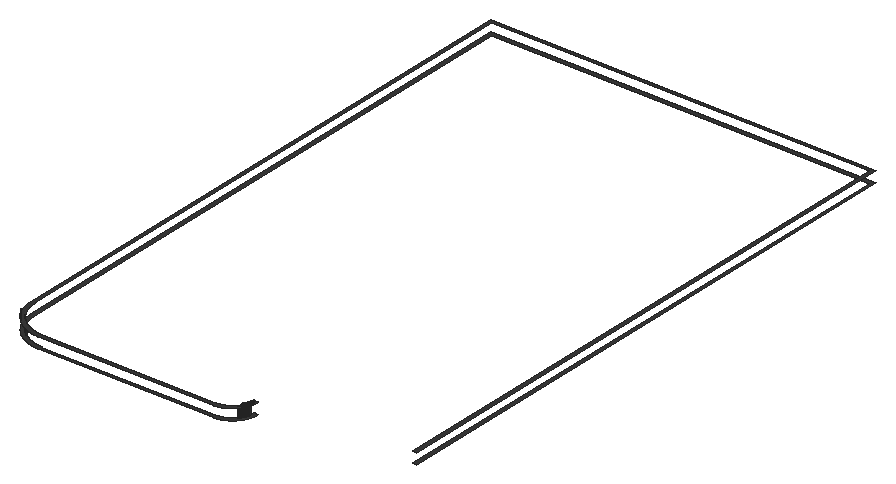
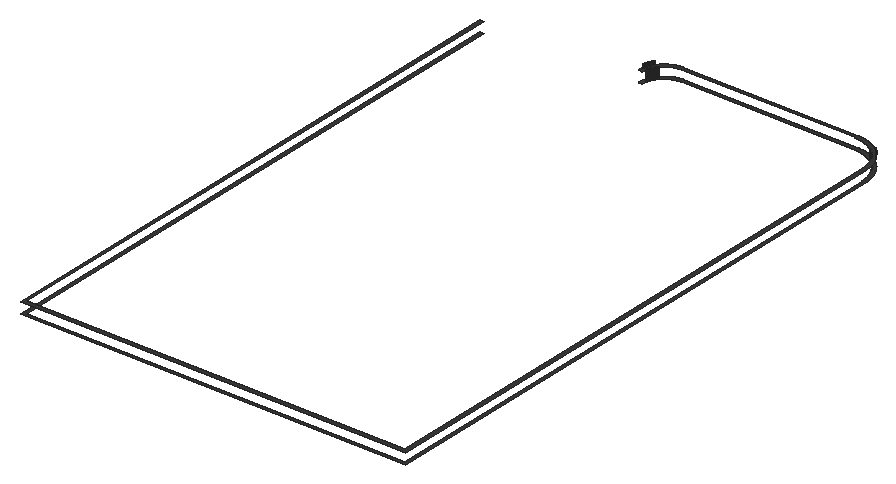
# SketchUp Ruby script. Lengths in inches.
U = 1.inch
M = Sketchup.active_model
def pt(a) = Geom::Point3d.new(a.map { |v| v * U })
def face(e, loops, mat)
  f = e.add_face(loops[0].map { |a| pt(a) })
  loops[1..].each { |l| e.add_face(l.map { |a| pt(a) }).erase! }
  f.material = f.back_material = mat if mat
  f
end
# faces: each face lists its corners as indices into pts; further lists are holes
def faces(e, pts, list, mat = nil) = list.each { |f| face(e, (f[0].is_a?(Array) ? f : [f]).map { |l| l.map { |i| pts[i] } }, mat) }
# xy, xz, yz: faces in a plane at the given z, y or x. An outline is a flat list of corners, or four numbers for a rectangle; further outlines are holes
def ring(l) = l.size == 4 ? [[l[0], l[1]], [l[2], l[1]], [l[2], l[3]], [l[0], l[3]]] : l.each_slice(2).to_a
def flat(e, list, mat, &to3) = list.each { |f| face(e, (f[0].is_a?(Array) ? f : [f]).map { |l| ring(l).map { |u, v| to3.(u, v) } }, mat) }
def xy(e, z, list, mat = nil) = flat(e, list, mat) { |x, y| [x, y, z] }
def xz(e, y, list, mat = nil) = flat(e, list, mat) { |x, z| [x, y, z] }
def yz(e, x, list, mat = nil) = flat(e, list, mat) { |y, z| [x, y, z] }
def lines(e, pts, list) = list.each { |a, b| e.add_line(pt(pts[a]), pt(pts[b])) }
# prism: a flat outline (further loops are holes) pulled along v
def prism(e, loops, v, mat = nil)
  f = face(e, loops, mat); d = Geom::Vector3d.new(v.map { |x| x * U })
  f.pushpull(f.normal.samedirection?(d) ? d.length : -d.length)
end
def box(e, o, s, mat = nil) = prism(e, [[o, [o[0] + s[0], o[1], o[2]], [o[0] + s[0], o[1] + s[1], o[2]], [o[0], o[1] + s[1], o[2]]]], [0, 0, s[2]], mat)
def at(x, y, z, deg = 0) = Geom::Transformation.translation(pt([x, y, z])) * Geom::Transformation.rotation(ORIGIN, Z_AXIS, deg.degrees)
def axes(o, x, y, z) = Geom::Transformation.new([*x, 0, *y, 0, *z, 0, *pt(o).to_a, 1])
def part(name) = M.definitions.add(name)
# library, detail: a bought-in or finely detailed component or shape, given as its bounding box
def library(name, o, s) = part(name).tap { |d| box(d.entities, o, s) }
def detail(e, o, s) = box(e.add_group.entities, o, s)
def put(e, d, t, mat = nil) = e.add_instance(d, t).tap { |i| i.material = mat if mat }
def group(e, t, mat = nil) = e.add_group.tap { |g| g.transformation = t; g.material = mat if mat }.entities
root = M.entities
M.materials.add("1496 AP 8293 CARBON COPY").color = [58, 58, 58]
xy(root,261,[[43.57,64,185.27,64,185.55,64.01,185.82,64.02,186.1,64.03,186.375,64.04,186.65,64.06,186.92,64.09,187.2,64.12,187.74,64.18,188.01,64.22,188.29,64.26,188.56,64.3,189.1,64.4,189.37,64.46,189.63,64.52,189.9,64.58,190.44,64.72,190.96,64.86,191.23,64.94,191.49,65.03,191.75,65.11,192.01,65.2,192.27,65.3,192.53,65.39,192.78,65.49,193.04,65.6,193.79,65.93,194.29,66.17,194.53,66.29,194.78,66.42,195.02,66.54,195.26,66.68,195.5,66.8125,195.74,66.95,195.97,67.09,196.21,67.24,196.4375,67.39,196.67,67.54,196.89,67.69,197.12,67.85,197.56,68.17,198.22,68.68,198.43,68.85,198.85,69.21,199.05,69.39,199.25,69.58,199.46,69.77,199.65,69.96,199.85,70.15,200.04,70.35,200.23,70.54,200.42,70.75,200.61,70.95,200.79,71.15,201.15,71.57,201.32,71.78,201.83,72.44,202.15,72.88,202.31,73.11,202.46,73.33,202.61,73.5625,202.76,73.79,202.91,74.03,203.05,74.26,203.1875,74.5,203.32,74.74,203.46,74.98,203.58,75.22,203.71,75.47,203.83,75.71,204.07,76.21,204.4,76.96,204.51,77.22,204.61,77.47,204.7,77.73,204.8,77.99,204.89,78.25,204.97,78.51,205.06,78.77,205.14,79.04,205.28,79.56,205.42,80.1,205.48,80.37,205.54,80.63,205.6,80.9,205.7,81.44,205.74,81.71,205.78,81.99,205.82,82.26,205.88,82.8,205.91,83.08,205.94,83.35,205.96,83.625,205.97,83.9,205.98,84.18,205.99,84.45,206,84.73,206,85,203,85,203,84.76,202.99,84.53,202.99,84.29,202.98,84.06,202.96,83.82,202.94,83.59,202.92,83.35,202.9,83.12,202.875,82.88,202.85,82.65,202.8125,82.42,202.78,82.18,202.7,81.72,202.65,81.49,202.61,81.26,202.56,81.03,202.5,80.8,202.45,80.57,202.39,80.34,202.32,80.11,202.26,79.89,202.19,79.66,202.12,79.4375,202.04,79.21,201.97,78.99,201.89,78.77,201.8,78.55,201.72,78.33,201.54,77.89,201.44,77.68,201.35,77.46,201.25,77.25,201.14,77.04,201.04,76.83,200.82,76.41,200.7,76.2,200.59,76,200.35,75.6,200.22,75.39,200.1,75.2,199.97,75,199.83,74.8,199.7,74.61,199.5625,74.42,199.42,74.23,199.28,74.04,199.14,73.86,198.99,73.67,198.84,73.49,198.6875,73.31,198.53,73.13,198.375,72.96,198.22,72.78,198.06,72.61,197.89,72.44,197.73,72.27,197.56,72.11,197.39,71.94,197.22,71.78,197.04,71.625,196.87,71.47,196.69,71.3125,196.51,71.16,196.33,71.01,196.14,70.86,195.96,70.72,195.77,70.58,195.58,70.4375,195.39,70.3,195.2,70.17,195,70.03,194.8,69.9,194.61,69.78,194.4,69.65,194,69.41,193.8,69.3,193.59,69.18,193.17,68.96,192.96,68.86,192.75,68.75,192.54,68.65,192.32,68.56,192.11,68.46,191.67,68.28,191.45,68.2,191.23,68.11,191.01,68.03,190.79,67.96,190.5625,67.88,190.34,67.81,190.11,67.74,189.89,67.68,189.66,67.61,189.43,67.55,189.2,67.5,188.97,67.44,188.74,67.39,188.51,67.35,188.28,67.3,187.82,67.22,187.58,67.1875,187.35,67.15,187.12,67.125,186.88,67.1,186.65,67.08,186.41,67.06,186.18,67.04,185.94,67.02,185.71,67.01,185.47,67.01,185.24,67,43.61,67,43.21,67.01,42.82,67.02,42.43,67.04,42.04,67.0625,41.65,67.09,41.25,67.125,40.86,67.16,40.08,67.26,39.7,67.31,38.92,67.43,38.53,67.5,38.15,67.58,37.76,67.66,37.38,67.74,36.62,67.92,36.24,68.02,35.86,68.125,35.48,68.24,35.1,68.35,34.36,68.59,33.62,68.85,33.25,68.99,32.88,69.14,32.52,69.28,32.16,69.4375,31.8,69.59,31.44,69.76,31.08,69.92,30.73,70.09,30.03,70.45,29.69,70.64,29.34,70.83,29,71.02,28.66,71.22,28.33,71.42,27.99,71.63,27.66,71.84,27.33,72.06,27.01,72.28,26.6875,72.5,26.37,72.73,26.05,72.96,25.43,73.44,25.12,73.6875,24.82,73.93,24.52,74.1875,24.22,74.44,23.93,74.71,23.64,74.97,23.35,75.24,23.07,75.51,22.51,76.07,22.24,76.35,21.97,76.64,21.71,76.93,21.44,77.22,21.1875,77.52,20.93,77.82,20.6875,78.12,20.44,78.43,19.96,79.05,19.73,79.37,19.5,79.6875,19.28,80.01,19.06,80.33,18.84,80.66,18.63,80.99,18.42,81.33,18.22,81.66,18.02,82,17.83,82.34,17.64,82.69,17.45,83.03,17.09,83.73,16.92,84.08,16.76,84.44,16.59,84.8,16.4375,85.16,16.28,85.52,16.14,85.88,15.99,86.25,15.85,86.62,15.59,87.36,15.35,88.1,15.24,88.48,15.125,88.86,15.02,89.24,14.92,89.62,14.74,90.38,14.66,90.76,14.58,91.15,14.5,91.53,14.43,91.92,14.31,92.7,14.26,93.08,14.16,93.86,14.125,94.25,14.09,94.65,14.0625,95.04,14.04,95.43,14.02,95.82,14.01,96.21,14,96.61,14,564,323,564,323,97,326,97,326,567,11,567,11,96.57,11.01,96.14,11.03,95.7,11.07,94.84,11.1,94.41,11.18,93.55,11.28,92.69,11.34,92.26,11.41,91.84,11.48,91.41,11.55,90.99,11.63,90.5625,11.72,90.14,11.8125,89.72,11.91,89.3,12.02,88.875,12.125,88.46,12.24,88.04,12.36,87.63,12.48,87.21,12.62,86.8,12.75,86.39,12.89,85.98,13.04,85.58,13.19,85.17,13.51,84.37,13.68,83.97,13.85,83.58,14.03,83.18,14.21,82.79,14.4,82.4,14.6,82.02,14.8,81.63,15,81.25,15.42,80.5,15.86,79.76,16.09,79.39,16.32,79.03,16.5625,78.67,16.8,78.31,17.05,77.95,17.3,77.6,17.56,77.26,17.82,76.91,18.08,76.57,18.35,76.23,18.91,75.57,19.1875,75.24,19.48,74.92,19.77,74.6,20.0625,74.28,20.36,73.97,20.67,73.67,20.97,73.36,21.28,73.0625,21.6,72.77,21.92,72.48,22.24,72.1875,22.57,71.91,23.23,71.35,23.57,71.08,23.91,70.82,24.26,70.56,24.6,70.3,24.95,70.05,25.31,69.8,25.67,69.5625,26.03,69.32,26.39,69.09,26.76,68.86,27.5,68.42,28.25,68,28.63,67.8,29.02,67.6,29.4,67.4,29.79,67.21,30.18,67.03,30.58,66.85,30.97,66.68,31.37,66.51,32.17,66.19,32.58,66.04,32.98,65.89,33.39,65.75,33.8,65.62,34.21,65.48,34.63,65.36,35.04,65.24,35.46,65.125,35.875,65.02,36.3,64.91,36.72,64.8125,37.14,64.72,37.5625,64.63,37.99,64.55,38.41,64.48,38.84,64.41,39.26,64.34,39.69,64.28,40.55,64.18,41.41,64.1,41.84,64.07,42.7,64.03,43.14,64.01]],"1496 AP 8293 CARBON COPY")
xy(root,270,[[43.57,64,43.14,64.01,42.7,64.03,41.84,64.07,41.41,64.1,40.55,64.18,39.69,64.28,39.26,64.34,38.84,64.41,38.41,64.48,37.99,64.55,37.5625,64.63,37.14,64.72,36.72,64.8125,36.3,64.91,35.875,65.02,35.46,65.125,35.04,65.24,34.63,65.36,34.21,65.48,33.8,65.62,33.39,65.75,32.98,65.89,32.58,66.04,32.17,66.19,31.37,66.51,30.97,66.68,30.58,66.85,30.18,67.03,29.79,67.21,29.4,67.4,29.02,67.6,28.63,67.8,28.25,68,27.5,68.42,26.76,68.86,26.39,69.09,26.03,69.32,25.67,69.5625,25.31,69.8,24.95,70.05,24.6,70.3,24.26,70.56,23.91,70.82,23.57,71.08,23.23,71.35,22.57,71.91,22.24,72.1875,21.92,72.48,21.6,72.77,21.28,73.0625,20.97,73.36,20.67,73.67,20.36,73.97,20.0625,74.28,19.77,74.6,19.48,74.92,19.1875,75.24,18.91,75.57,18.35,76.23,18.08,76.57,17.82,76.91,17.56,77.26,17.3,77.6,17.05,77.95,16.8,78.31,16.5625,78.67,16.32,79.03,16.09,79.39,15.86,79.76,15.42,80.5,15,81.25,14.8,81.63,14.6,82.02,14.4,82.4,14.21,82.79,14.03,83.18,13.85,83.58,13.68,83.97,13.51,84.37,13.19,85.17,13.04,85.58,12.89,85.98,12.75,86.39,12.62,86.8,12.48,87.21,12.36,87.63,12.24,88.04,12.125,88.46,12.02,88.875,11.91,89.3,11.8125,89.72,11.72,90.14,11.63,90.5625,11.55,90.99,11.48,91.41,11.41,91.84,11.34,92.26,11.28,92.69,11.18,93.55,11.1,94.41,11.07,94.84,11.03,95.7,11.01,96.14,11,96.57,11,567,326,567,326,97,323,97,323,564,14,564,14,96.61,14.01,96.21,14.02,95.82,14.04,95.43,14.0625,95.04,14.09,94.65,14.125,94.25,14.16,93.86,14.26,93.08,14.31,92.7,14.43,91.92,14.5,91.53,14.58,91.15,14.66,90.76,14.74,90.38,14.92,89.62,15.02,89.24,15.125,88.86,15.24,88.48,15.35,88.1,15.59,87.36,15.85,86.62,15.99,86.25,16.14,85.88,16.28,85.52,16.4375,85.16,16.59,84.8,16.76,84.44,16.92,84.08,17.09,83.73,17.45,83.03,17.64,82.69,17.83,82.34,18.02,82,18.22,81.66,18.42,81.33,18.63,80.99,18.84,80.66,19.06,80.33,19.28,80.01,19.5,79.6875,19.73,79.37,19.96,79.05,20.44,78.43,20.6875,78.12,20.93,77.82,21.1875,77.52,21.44,77.22,21.71,76.93,21.97,76.64,22.24,76.35,22.51,76.07,23.07,75.51,23.35,75.24,23.64,74.97,23.93,74.71,24.22,74.44,24.52,74.1875,24.82,73.93,25.12,73.6875,25.43,73.44,26.05,72.96,26.37,72.73,26.6875,72.5,27.01,72.28,27.33,72.06,27.66,71.84,27.99,71.63,28.33,71.42,28.66,71.22,29,71.02,29.34,70.83,29.69,70.64,30.03,70.45,30.73,70.09,31.08,69.92,31.44,69.76,31.8,69.59,32.16,69.4375,32.52,69.28,32.88,69.14,33.25,68.99,33.62,68.85,34.36,68.59,35.1,68.35,35.48,68.24,35.86,68.125,36.24,68.02,36.62,67.92,37.38,67.74,37.76,67.66,38.15,67.58,38.53,67.5,38.92,67.43,39.7,67.31,40.08,67.26,40.86,67.16,41.25,67.125,41.65,67.09,42.04,67.0625,42.43,67.04,42.82,67.02,43.21,67.01,43.61,67,185.24,67,185.47,67.01,185.71,67.01,185.94,67.02,186.18,67.04,186.41,67.06,186.65,67.08,186.88,67.1,187.12,67.125,187.35,67.15,187.58,67.1875,187.82,67.22,188.28,67.3,188.51,67.35,188.74,67.39,188.97,67.44,189.2,67.5,189.43,67.55,189.66,67.61,189.89,67.68,190.11,67.74,190.34,67.81,190.5625,67.88,190.79,67.96,191.01,68.03,191.23,68.11,191.45,68.2,191.67,68.28,192.11,68.46,192.32,68.56,192.54,68.65,192.75,68.75,192.96,68.86,193.17,68.96,193.59,69.18,193.8,69.3,194,69.41,194.4,69.65,194.61,69.78,194.8,69.9,195,70.03,195.2,70.17,195.39,70.3,195.58,70.4375,195.77,70.58,195.96,70.72,196.14,70.86,196.33,71.01,196.51,71.16,196.69,71.3125,196.87,71.47,197.04,71.625,197.22,71.78,197.39,71.94,197.56,72.11,197.73,72.27,197.89,72.44,198.06,72.61,198.22,72.78,198.375,72.96,198.53,73.13,198.6875,73.31,198.84,73.49,198.99,73.67,199.14,73.86,199.28,74.04,199.42,74.23,199.5625,74.42,199.7,74.61,199.83,74.8,199.97,75,200.1,75.2,200.22,75.39,200.35,75.6,200.59,76,200.7,76.2,200.82,76.41,201.04,76.83,201.14,77.04,201.25,77.25,201.35,77.46,201.44,77.68,201.54,77.89,201.72,78.33,201.8,78.55,201.89,78.77,201.97,78.99,202.04,79.21,202.12,79.4375,202.19,79.66,202.26,79.89,202.32,80.11,202.39,80.34,202.45,80.57,202.5,80.8,202.56,81.03,202.61,81.26,202.65,81.49,202.7,81.72,202.78,82.18,202.8125,82.42,202.85,82.65,202.875,82.88,202.9,83.12,202.92,83.35,202.94,83.59,202.96,83.82,202.98,84.06,202.99,84.29,202.99,84.53,203,84.76,203,85,206,85,206,84.73,205.99,84.45,205.98,84.18,205.97,83.9,205.96,83.625,205.94,83.35,205.91,83.08,205.88,82.8,205.82,82.26,205.78,81.99,205.74,81.71,205.7,81.44,205.6,80.9,205.54,80.63,205.48,80.37,205.42,80.1,205.28,79.56,205.14,79.04,205.06,78.77,204.97,78.51,204.89,78.25,204.8,77.99,204.7,77.73,204.61,77.47,204.51,77.22,204.4,76.96,204.07,76.21,203.83,75.71,203.71,75.47,203.58,75.22,203.46,74.98,203.32,74.74,203.1875,74.5,203.05,74.26,202.91,74.03,202.76,73.79,202.61,73.5625,202.46,73.33,202.31,73.11,202.15,72.88,201.83,72.44,201.32,71.78,201.15,71.57,200.79,71.15,200.61,70.95,200.42,70.75,200.23,70.54,200.04,70.35,199.85,70.15,199.65,69.96,199.46,69.77,199.25,69.58,199.05,69.39,198.85,69.21,198.43,68.85,198.22,68.68,197.56,68.17,197.12,67.85,196.89,67.69,196.67,67.54,196.4375,67.39,196.21,67.24,195.97,67.09,195.74,66.95,195.5,66.8125,195.26,66.68,195.02,66.54,194.78,66.42,194.53,66.29,194.29,66.17,193.79,65.93,193.04,65.6,192.78,65.49,192.53,65.39,192.27,65.3,192.01,65.2,191.75,65.11,191.49,65.03,191.23,64.94,190.96,64.86,190.44,64.72,189.9,64.58,189.63,64.52,189.37,64.46,189.1,64.4,188.56,64.3,188.29,64.26,188.01,64.22,187.74,64.18,187.2,64.12,186.92,64.09,186.65,64.06,186.375,64.04,186.1,64.03,185.82,64.02,185.55,64.01,185.27,64]],"1496 AP 8293 CARBON COPY")
p = [[198.6875,73.31,261],[198.6875,73.31,270],[198.53,73.13,270],[198.53,73.13,261],[25.74,73.2,261],[25.74,73.2,270],
  [25.43,73.44,270],[25.43,73.44,261],[198.84,73.49,261],[198.84,73.49,270],[25.12,73.6875,270],[25.12,73.6875,261],
  [198.99,73.67,261],[198.99,73.67,270],[24.82,73.93,270],[24.82,73.93,261],[199.14,73.86,261],[199.14,73.86,270],
  [24.52,74.1875,270],[24.52,74.1875,261],[199.28,74.04,261],[199.28,74.04,270],[199.42,74.23,261],[199.42,74.23,270],
  [24.22,74.44,270],[24.22,74.44,261],[199.5625,74.42,261],[199.5625,74.42,270],[23.93,74.71,270],[23.93,74.71,261],
  [199.7,74.61,261],[199.7,74.61,270],[199.83,74.8,261],[199.83,74.8,270],[23.64,74.97,270],[23.64,74.97,261],
  [199.97,75,261],[199.97,75,270],[23.35,75.24,270],[23.35,75.24,261],[200.1,75.2,261],[200.1,75.2,270],
  [23.07,75.51,270],[23.07,75.51,261],[200.22,75.39,261],[200.22,75.39,270],[200.35,75.6,261],[200.35,75.6,270],
  [22.79,75.79,270],[22.79,75.79,261],[200.47,75.8,261],[200.47,75.8,270],[22.51,76.07,270],[22.51,76.07,261],
  [200.59,76,261],[200.59,76,270],[200.7,76.2,261],[200.7,76.2,270],[22.24,76.35,270],[22.24,76.35,261],
  [200.82,76.41,261],[200.82,76.41,270],[21.97,76.64,270],[21.97,76.64,261],[200.93,76.62,261],[200.93,76.62,270],
  [21.71,76.93,270],[21.71,76.93,261],[201.04,76.83,261],[201.04,76.83,270],[201.14,77.04,261],[201.14,77.04,270],
  [21.44,77.22,270],[21.44,77.22,261],[201.25,77.25,261],[201.25,77.25,270],[21.1875,77.52,270],[21.1875,77.52,261],
  [201.35,77.46,261],[201.35,77.46,270],[20.93,77.82,270],[20.93,77.82,261],[201.44,77.68,261],[201.44,77.68,270],
  [201.54,77.89,261],[201.54,77.89,270],[20.6875,78.12,270],[20.6875,78.12,261],[201.63,78.11,261],[201.63,78.11,270],
  [20.44,78.43,270],[20.44,78.43,261],[201.72,78.33,261],[201.72,78.33,270],[201.8,78.55,261],[201.8,78.55,270],
  [20.2,78.74,270],[20.2,78.74,261],[201.89,78.77,261],[201.89,78.77,270],[19.96,79.05,270],[19.96,79.05,261],
  [201.97,78.99,261],[201.97,78.99,270],[202.04,79.21,261],[202.04,79.21,270],[19.73,79.37,270],[19.73,79.37,261],
  [202.12,79.4375,261],[202.12,79.4375,270],[19.5,79.6875,270],[19.5,79.6875,261],[202.19,79.66,261],[202.19,79.66,270],
  [19.28,80.01,270],[19.28,80.01,261],[202.26,79.89,261],[202.26,79.89,270],[202.32,80.11,261],[202.32,80.11,270],
  [19.06,80.33,270],[19.06,80.33,261],[202.39,80.34,261],[202.39,80.34,270],[18.84,80.66,270],[18.84,80.66,261],
  [202.45,80.57,261],[202.45,80.57,270],[202.5,80.8,261],[202.5,80.8,270],[18.63,80.99,270],[18.63,80.99,261],
  [202.56,81.03,261],[202.56,81.03,270],[202.61,81.26,261],[202.61,81.26,270],[20.97,73.36,270],[21.28,73.0625,270],
  [21.28,73.0625,273],[20.97,73.36,273],[202.31,73.11,270],[202.46,73.33,270],[202.46,73.33,273],[202.31,73.11,273],
  [202.61,73.5625,270],[202.61,73.5625,273],[20.67,73.67,270],[20.67,73.67,273],[202.76,73.79,270],[202.76,73.79,273],
  [20.36,73.97,270],[20.36,73.97,273],[202.91,74.03,270],[202.91,74.03,273],[20.0625,74.28,270],[20.0625,74.28,273],
  [203.05,74.26,270],[203.05,74.26,273],[19.77,74.6,270],[19.77,74.6,273],[203.1875,74.5,270],[203.1875,74.5,273],
  [203.32,74.74,270],[203.32,74.74,273],[19.48,74.92,270],[19.48,74.92,273],[203.46,74.98,270],[203.46,74.98,273],
  [19.1875,75.24,270],[19.1875,75.24,273],[203.58,75.22,270],[203.58,75.22,273],[18.91,75.57,270],[18.91,75.57,273],
  [203.71,75.47,270],[203.71,75.47,273],[203.83,75.71,270],[203.83,75.71,273],[18.63,75.9,270],[18.63,75.9,273],
  [203.95,75.96,270],[203.95,75.96,273],[18.35,76.23,270],[18.35,76.23,273],[204.07,76.21,270],[204.07,76.21,273],
  [18.08,76.57,270],[18.08,76.57,273],[204.18,76.46,270],[204.18,76.46,273],[204.29,76.71,270],[204.29,76.71,273],
  [17.82,76.91,270],[17.82,76.91,273],[204.4,76.96,270],[204.4,76.96,273],[17.56,77.26,270],[17.56,77.26,273],
  [204.51,77.22,270],[204.51,77.22,273],[204.61,77.47,270],[204.61,77.47,273],[17.3,77.6,270],[17.3,77.6,273],
  [204.7,77.73,270],[204.7,77.73,273],[17.05,77.95,270],[17.05,77.95,273],[204.8,77.99,270],[204.8,77.99,273],
  [16.8,78.31,270],[16.8,78.31,273],[204.89,78.25,270],[204.89,78.25,273],[204.97,78.51,270],[204.97,78.51,273],
  [16.5625,78.67,270],[16.5625,78.67,273],[205.06,78.77,270],[205.06,78.77,273],[16.32,79.03,270],[16.32,79.03,273],
  [205.14,79.04,270],[205.14,79.04,273],[16.09,79.39,270],[16.09,79.39,273],[205.21,79.3,270],[205.21,79.3,273],
  [205.28,79.56,270],[205.28,79.56,273],[15.86,79.76,270],[15.86,79.76,273],[205.35,79.83,270],[205.35,79.83,273],
  [15.64,80.13,270],[15.64,80.13,273],[205.42,80.1,270],[205.42,80.1,273],[15.42,80.5,270],[15.42,80.5,273],
  [205.48,80.37,270],[205.48,80.37,273],[205.54,80.63,270],[205.54,80.63,273],[15.21,80.875,270],[15.21,80.875,273],
  [205.6,80.9,270],[205.6,80.9,273],[15,81.25,270],[15,81.25,273],[205.65,81.17,270],[205.65,81.17,273]]
faces(root,p,[[0,1,2,3],[4,5,6,7],[8,9,1,0],[7,6,10,11],[12,13,9,8],[11,10,14,15],[16,17,13,12],[15,14,18,19],
  [20,21,17,16],[22,23,21,20],[19,18,24,25],[26,27,23,22],[25,24,28,29],[30,31,27,26],[32,33,31,30],[29,28,34,35],
  [36,37,33,32],[35,34,38,39],[40,41,37,36],[39,38,42,43],[44,45,41,40],[46,47,45,44],[43,42,48,49],[50,51,47,46],
  [49,48,52,53],[54,55,51,50],[56,57,55,54],[53,52,58,59],[60,61,57,56],[59,58,62,63],[64,65,61,60],[63,62,66,67],
  [68,69,65,64],[70,71,69,68],[67,66,72,73],[74,75,71,70],[73,72,76,77],[78,79,75,74],[77,76,80,81],[82,83,79,78],
  [84,85,83,82],[81,80,86,87],[88,89,85,84],[87,86,90,91],[92,93,89,88],[94,95,93,92],[91,90,96,97],[98,99,95,94],
  [97,96,100,101],[102,103,99,98],[104,105,103,102],[101,100,106,107],[108,109,105,104],[107,106,110,111],[112,113,109,108],[111,110,114,115],
  [116,117,113,112],[118,119,117,116],[115,114,120,121],[122,123,119,118],[121,120,124,125],[126,127,123,122],[128,129,127,126],[125,124,130,131],
  [132,133,129,128],[134,135,133,132],[136,137,138,139],[140,141,142,143],[141,144,145,142],[146,136,139,147],[144,148,149,145],[150,146,147,151],
  [148,152,153,149],[154,150,151,155],[152,156,157,153],[158,154,155,159],[156,160,161,157],[160,162,163,161],[164,158,159,165],[162,166,167,163],
  [168,164,165,169],[166,170,171,167],[172,168,169,173],[170,174,175,171],[174,176,177,175],[178,172,173,179],[176,180,181,177],[182,178,179,183],
  [180,184,185,181],[186,182,183,187],[184,188,189,185],[188,190,191,189],[192,186,187,193],[190,194,195,191],[196,192,193,197],[194,198,199,195],
  [198,200,201,199],[202,196,197,203],[200,204,205,201],[206,202,203,207],[204,208,209,205],[210,206,207,211],[208,212,213,209],[212,214,215,213],
  [216,210,211,217],[214,218,219,215],[220,216,217,221],[218,222,223,219],[224,220,221,225],[222,226,227,223],[226,228,229,227],[230,224,225,231],
  [228,232,233,229],[234,230,231,235],[232,236,237,233],[238,234,235,239],[236,240,241,237],[240,242,243,241],[244,238,239,245],[242,246,247,243],
  [248,244,245,249],[246,250,251,247]],"1496 AP 8293 CARBON COPY")
